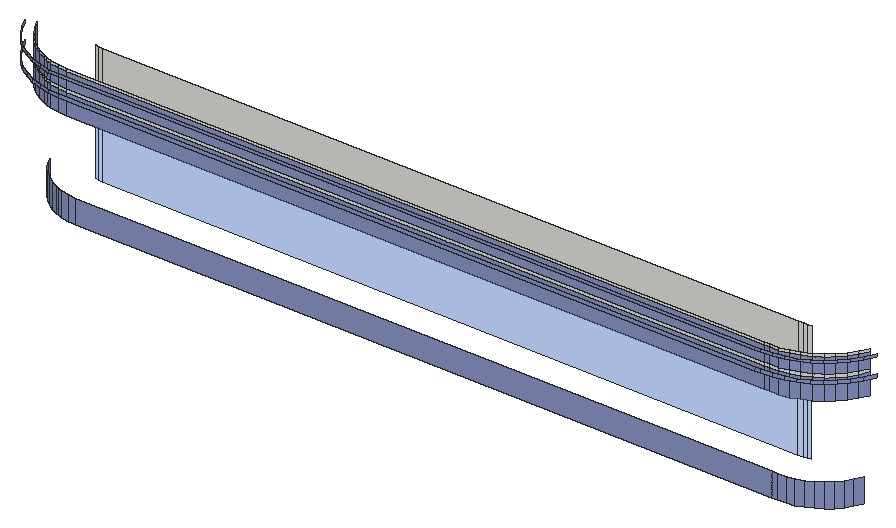
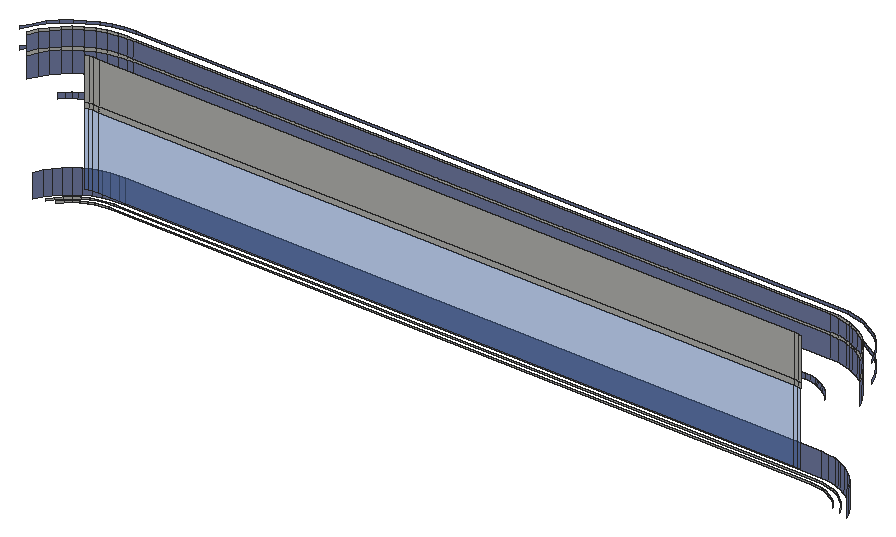
# SketchUp Ruby script. Lengths in inches.
U = 1.inch
M = Sketchup.active_model
def pt(a) = Geom::Point3d.new(a.map { |v| v * U })
def face(e, loops, mat)
  f = e.add_face(loops[0].map { |a| pt(a) })
  loops[1..].each { |l| e.add_face(l.map { |a| pt(a) }).erase! }
  f.material = f.back_material = mat if mat
  f
end
# faces: each face lists its corners as indices into pts; further lists are holes
def faces(e, pts, list, mat = nil) = list.each { |f| face(e, (f[0].is_a?(Array) ? f : [f]).map { |l| l.map { |i| pts[i] } }, mat) }
# xy, xz, yz: faces in a plane at the given z, y or x. An outline is a flat list of corners, or four numbers for a rectangle; further outlines are holes
def ring(l) = l.size == 4 ? [[l[0], l[1]], [l[2], l[1]], [l[2], l[3]], [l[0], l[3]]] : l.each_slice(2).to_a
def flat(e, list, mat, &to3) = list.each { |f| face(e, (f[0].is_a?(Array) ? f : [f]).map { |l| ring(l).map { |u, v| to3.(u, v) } }, mat) }
def xy(e, z, list, mat = nil) = flat(e, list, mat) { |x, y| [x, y, z] }
def xz(e, y, list, mat = nil) = flat(e, list, mat) { |x, z| [x, y, z] }
def yz(e, x, list, mat = nil) = flat(e, list, mat) { |y, z| [x, y, z] }
def lines(e, pts, list) = list.each { |a, b| e.add_line(pt(pts[a]), pt(pts[b])) }
# prism: a flat outline (further loops are holes) pulled along v
def prism(e, loops, v, mat = nil)
  f = face(e, loops, mat); d = Geom::Vector3d.new(v.map { |x| x * U })
  f.pushpull(f.normal.samedirection?(d) ? d.length : -d.length)
end
def box(e, o, s, mat = nil) = prism(e, [[o, [o[0] + s[0], o[1], o[2]], [o[0] + s[0], o[1] + s[1], o[2]], [o[0], o[1] + s[1], o[2]]]], [0, 0, s[2]], mat)
def at(x, y, z, deg = 0) = Geom::Transformation.translation(pt([x, y, z])) * Geom::Transformation.rotation(ORIGIN, Z_AXIS, deg.degrees)
def axes(o, x, y, z) = Geom::Transformation.new([*x, 0, *y, 0, *z, 0, *pt(o).to_a, 1])
def part(name) = M.definitions.add(name)
# library, detail: a bought-in or finely detailed component or shape, given as its bounding box
def library(name, o, s) = part(name).tap { |d| box(d.entities, o, s) }
def detail(e, o, s) = box(e.add_group.entities, o, s)
def put(e, d, t, mat = nil) = e.add_instance(d, t).tap { |i| i.material = mat if mat }
def group(e, t, mat = nil) = e.add_group.tap { |g| g.transformation = t; g.material = mat if mat }.entities
root = M.entities
M.materials.add("0326 AP 7207 CLASSIC PURPLE").color = [140, 152, 201]
M.materials.add("[Translucent Glass Blue]").color = [100, 149, 237]
M.materials["[Translucent Glass Blue]"].alpha = 0.5
xz(root,31.9,[[167.34,433.9375,517.41,435.625],[517.41,433.9375,520.4375,435.625],[167.34,443.3125,517.41,444.625],[517.41,443.3125,520.4375,444.625]],"0326 AP 7207 CLASSIC PURPLE")
xz(root,37.02,[[167.51,433.9375,517.41,435.625],[517.41,433.9375,520.4375,435.625],[167.51,443.3125,517.41,444.625],[517.41,443.3125,520.4375,444.625]])
xz(root,37.02,[[167.51,423.4375,517.41,433.9375],[517.41,423.4375,520.4375,433.9375],[167.51,435.625,517.41,443.3125],[517.41,435.625,520.4375,443.3125]],"0326 AP 7207 CLASSIC PURPLE")
xz(root,42.4375,[[167.6875,372,517.41,384],[517.41,372,520.4375,384]],"0326 AP 7207 CLASSIC PURPLE")
xz(root,45.71,[[167.8,372,517.41,372.8125],[517.41,372,520.4375,372.8125]])
xz(root,48.77,[[167.9,372,517.41,372.8125],[517.41,372,520.4375,372.8125]])
xz(root,52.13,[[168.01,420.75,517.41,423.4375],[517.41,420.75,520.4375,423.4375]],"0326 AP 7207 CLASSIC PURPLE")
xz(root,58.64,[[168.22,420.75,517.41,423.4375],[517.41,420.75,520.4375,423.4375],[168.22,423.4375,517.41,444.625],[517.41,423.4375,520.4375,444.625]])
xz(root,58.64,[[168.22,384,517.41,420.75],[517.41,384,520.4375,420.75]],"[Translucent Glass Blue]")
p = [[167.6875,42.4375,384],[163.74,42.7,384],[163.74,42.7,372],[166.41,42.52,372],[167.6875,42.4375,372],[524.38,42.7,384],
  [520.4375,42.4375,384],[520.4375,42.4375,372],[524.38,42.7,372],[159.87,43.47,384],[159.87,43.47,372],[528.26,43.47,384],
  [528.26,43.47,372],[157.41,44.3,384],[157.41,44.3,372],[532,44.74,384],[532,44.74,372],[156.125,44.74,384],
  [156.125,44.74,372],[152.58,46.49,384],[152.58,46.49,372],[535.55,46.49,384],[535.55,46.49,372],[167.8,45.71,372],
  [166.62,45.78,372],[166.62,45.78,372.8125],[167.8,45.71,372.8125],[523.96,45.9375,372],[520.4375,45.71,372],[520.4375,45.71,372.8125],
  [523.96,45.9375,372.8125],[164.17,45.95,372],[164.17,45.95,372.8125],[160.72,46.63,372],[160.72,46.63,372.8125],[527.41,46.625,372],
  [527.41,46.625,372.8125],[149.29,48.68,384],[149.29,48.68,372],[538.83,48.68,384],[538.83,48.68,372],[158.46,47.4,372],
  [158.46,47.4,372.8125],[530.75,47.76,372],[530.75,47.76,372.8125],[157.38,47.77,372],[157.38,47.77,372.8125],[154.22,49.32,372],
  [154.22,49.32,372.8125],[533.91,49.32,372],[533.91,49.32,372.8125],[146.32,51.29,384],[146.32,51.29,372],[541.81,51.29,384],
  [541.81,51.29,372],[164.57,48.98,372],[166.82,48.84,372],[166.82,48.84,372.8125],[164.57,48.98,372.8125],[167.9,48.77,372],
  [167.9,48.77,372.8125],[520.4375,48.77,372],[523.56,48.97,372],[523.56,48.97,372.8125],[520.4375,48.77,372.8125],[161.51,49.59,372],
  [161.51,49.59,372.8125],[526.62,49.58,372],[526.62,49.58,372.8125],[151.29,51.28,372],[151.29,51.28,372.8125],[536.84,51.28,372],
  [536.84,51.28,372.8125],[159.44,50.3,372],[159.44,50.3,372.8125],[529.58,50.59,372],[529.58,50.59,372.8125],[158.55,50.6,372],
  [158.55,50.6,372.8125],[155.75,51.98,372],[155.75,51.98,372.8125],[532.38,51.97,372],[532.38,51.97,372.8125],[143.71,54.26,384],
  [143.71,54.26,372],[148.64,53.61,372],[148.64,53.61,372.8125],[539.49,53.6,372],[539.49,53.6,372.8125],[544.41,54.26,384],
  [544.41,54.26,372],[153.15,53.71,372],[153.15,53.71,372.8125],[534.98,53.7,372],[534.98,53.7,372.8125],[146.3125,56.26,372],
  [146.3125,56.26,372.8125],[541.82,56.25,372],[541.82,56.25,372.8125],[150.81,55.77,372],[150.81,55.77,372.8125],[537.33,55.76,372],
  [537.33,55.76,372.8125],[141.52,57.55,384],[141.52,57.55,372],[546.61,57.55,384],[546.61,57.55,372],[148.75,58.12,372],
  [148.75,58.12,372.8125],[539.39,58.11,372],[539.39,58.11,372.8125],[144.36,59.1875,372],[144.36,59.1875,372.8125],[543.78,59.18,372],
  [543.78,59.18,372.8125],[139.77,61.09,384],[139.77,61.09,372],[548.36,61.09,384],[548.36,61.09,372],[165.86,58.8,384],
  [168.22,58.64,384],[168.22,58.64,420.75],[165.86,58.8,420.75],[520.4375,58.64,384],[522.27,58.76,384],[522.27,58.76,420.75],
  [520.4375,58.64,420.75],[164.07,59.15,384],[164.07,59.15,420.75],[524.06,59.12,384],[524.06,59.12,420.75],[168.01,52.13,423.4375],
  [165.01,52.33,423.4375],[165.01,52.33,420.75],[168.01,52.13,420.75],[523.12,52.31,423.4375],[520.4375,52.13,423.4375],[520.4375,52.13,420.75],
  [523.12,52.31,420.75],[162.38,52.85,423.4375],[162.38,52.85,420.75],[525.75,52.83,423.4375],[525.75,52.83,420.75],[528.29,53.7,423.4375],
  [528.29,53.7,420.75],[160.52,53.48,423.4375],[160.52,53.48,420.75],[159.84,53.72,423.4375],[159.84,53.72,420.75],[157.4375,54.9,423.4375],
  [157.4375,54.9,420.75],[530.7,54.88,423.4375],[530.7,54.88,420.75],[155.21,56.39,423.4375],[155.21,56.39,420.75],[532.93,56.375,423.4375],
  [532.93,56.375,420.75],[153.19,58.16,423.4375],[153.19,58.16,420.75],[534.95,58.15,423.4375],[534.95,58.15,420.75],[536.72,60.16,423.4375],
  [536.72,60.16,420.75],[151.42,60.18,423.4375],[151.42,60.18,420.75],[168.22,58.64,423.4375],[165.86,58.8,423.4375],[522.27,58.76,423.4375],
  [520.4375,58.64,423.4375],[164.07,59.15,423.4375],[524.06,59.12,423.4375],[163.03,37.3125,423.4375],[167.51,37.02,423.4375],[167.51,37.02,433.9375],
  [163.03,37.3125,433.9375],[520.4375,37.02,423.4375],[525.09,37.32,423.4375],[525.09,37.32,433.9375],[520.4375,37.02,433.9375],[158.46,38.22,423.4375],
  [158.46,38.22,433.9375],[529.66,38.23,423.4375],[529.66,38.23,433.9375],[155.67,39.17,423.4375],[155.67,39.17,433.9375],[534.08,39.73,423.4375],
  [534.08,39.73,433.9375],[154.05,39.72,423.4375],[154.05,39.72,433.9375],[149.86,41.78,423.4375],[149.86,41.78,433.9375],[538.26,41.79,423.4375],
  [538.26,41.79,433.9375],[145.99,44.375,423.4375],[145.99,44.375,433.9375],[542.13,44.38,423.4375],[542.13,44.38,433.9375],[142.48,47.45,423.4375],
  [142.48,47.45,433.9375],[545.64,47.46,423.4375],[545.64,47.46,433.9375],[139.41,50.95,423.4375],[139.41,50.95,433.9375],[548.71,50.96,423.4375],
  [548.71,50.96,433.9375],[136.82,54.83,423.4375],[136.82,54.83,433.9375],[551.3,54.84,423.4375],[551.3,54.84,433.9375],[134.75,59.01,423.4375],
  [134.75,59.01,433.9375],[553.36,59.02,423.4375],[553.36,59.02,433.9375],[165.86,58.8,444.625],[168.22,58.64,444.625],[520.4375,58.64,444.625],
  [522.27,58.76,444.625],[164.07,59.15,444.625],[524.06,59.12,444.625],[162.36,32.22,433.9375],[167.34,31.9,433.9375],[167.34,31.9,435.625],
  [162.36,32.22,435.625],[520.4375,31.9,433.9375],[525.76,32.24,433.9375],[525.76,32.24,435.625],[520.4375,31.9,435.625],[157.13,33.26,433.9375],
  [157.13,33.26,435.625],[530.99,33.28,433.9375],[530.99,33.28,435.625],[154.02,34.32,433.9375],[154.02,34.32,435.625],[536.04,35,433.9375],
  [536.04,35,435.625],[152.08,34.98,433.9375],[152.08,34.98,435.625],[147.3,37.34,433.9375],[147.3,37.34,435.625],[540.82,37.36,433.9375],
  [540.82,37.36,435.625],[163.03,37.3125,435.625],[167.51,37.02,435.625],[520.4375,37.02,435.625],[525.09,37.32,435.625],[142.86,40.3,433.9375],
  [142.86,40.3,435.625],[158.46,38.22,435.625],[529.66,38.23,435.625],[545.25,40.32,433.9375],[545.25,40.32,435.625],[155.67,39.17,435.625],
  [534.08,39.73,435.625],[154.05,39.72,435.625],[149.86,41.78,435.625],[538.26,41.79,435.625],[138.85,43.82,433.9375],[138.85,43.82,435.625],
  [549.26,43.83,433.9375],[549.26,43.83,435.625],[145.99,44.375,435.625],[542.13,44.38,435.625],[135.33,47.83,433.9375],[135.33,47.83,435.625],
  [552.78,47.84,433.9375],[552.78,47.84,435.625],[142.48,47.45,435.625],[545.64,47.46,435.625],[139.41,50.95,435.625],[548.71,50.96,435.625],
  [132.37,52.26,433.9375],[132.37,52.26,435.625],[555.74,52.28,433.9375],[555.74,52.28,435.625],[136.82,54.83,435.625],[551.3,54.84,435.625],
  [130.01,57.05,433.9375],[130.01,57.05,435.625],[558.1,57.06,433.9375],[558.1,57.06,435.625],[134.75,59.01,435.625],[553.36,59.02,435.625],
  [167.51,37.02,443.3125],[163.03,37.3125,443.3125],[525.09,37.32,443.3125],[520.4375,37.02,443.3125],[158.46,38.22,443.3125],[529.66,38.23,443.3125],
  [155.67,39.17,443.3125],[534.08,39.73,443.3125],[154.05,39.72,443.3125],[149.86,41.78,443.3125],[538.26,41.79,443.3125],[145.99,44.375,443.3125],
  [542.13,44.38,443.3125],[142.48,47.45,443.3125],[545.64,47.46,443.3125],[139.41,50.95,443.3125],[548.71,50.96,443.3125],[136.82,54.83,443.3125],
  [551.3,54.84,443.3125],[134.75,59.01,443.3125],[553.36,59.02,443.3125],[162.36,32.22,443.3125],[167.34,31.9,443.3125],[167.34,31.9,444.625],
  [162.36,32.22,444.625],[520.4375,31.9,443.3125],[525.76,32.24,443.3125],[525.76,32.24,444.625],[520.4375,31.9,444.625],[157.13,33.26,443.3125],
  [157.13,33.26,444.625],[530.99,33.28,443.3125],[530.99,33.28,444.625],[154.02,34.32,443.3125],[154.02,34.32,444.625],[536.04,35,443.3125],
  [536.04,35,444.625],[152.08,34.98,443.3125],[152.08,34.98,444.625],[147.3,37.34,443.3125],[147.3,37.34,444.625],[540.82,37.36,443.3125],
  [540.82,37.36,444.625],[163.03,37.3125,444.625],[167.51,37.02,444.625],[520.4375,37.02,444.625],[525.09,37.32,444.625],[142.86,40.3,443.3125],
  [142.86,40.3,444.625],[158.46,38.22,444.625],[529.66,38.23,444.625],[545.25,40.32,443.3125],[545.25,40.32,444.625],[155.67,39.17,444.625],
  [534.08,39.73,444.625],[154.05,39.72,444.625],[149.86,41.78,444.625],[538.26,41.79,444.625],[138.85,43.82,443.3125],[138.85,43.82,444.625],
  [549.26,43.83,443.3125],[549.26,43.83,444.625],[145.99,44.375,444.625],[542.13,44.38,444.625],[135.33,47.83,443.3125],[135.33,47.83,444.625],
  [552.78,47.84,443.3125],[552.78,47.84,444.625],[142.48,47.45,444.625],[545.64,47.46,444.625],[139.41,50.95,444.625],[548.71,50.96,444.625],
  [132.37,52.26,443.3125],[132.37,52.26,444.625],[555.74,52.28,443.3125],[555.74,52.28,444.625],[136.82,54.83,444.625],[551.3,54.84,444.625],
  [130.01,57.05,443.3125],[130.01,57.05,444.625],[558.1,57.06,443.3125],[558.1,57.06,444.625],[134.75,59.01,444.625],[553.36,59.02,444.625]]
faces(root,p,[[0,1,2,3,4],[5,6,7,8],[1,9,10,2],[11,5,8,12],[9,13,14,10],[15,11,12,16],[13,17,18,14],[17,19,20,18],
  [21,15,16,22],[19,37,38,20],[39,21,22,40],[37,51,52,38],[53,39,40,54],[51,83,84,52],[89,53,54,90],[83,103,104,84],
  [105,89,90,106],[103,115,116,104],[117,105,106,118],[131,132,133,134],[135,136,137,138],[132,139,140,133],[141,135,138,142],[143,141,142,144],
  [139,145,146,140],[145,147,148,146],[147,149,150,148],[151,143,144,152],[149,153,154,150],[155,151,152,156],[153,157,158,154],[159,155,156,160],
  [161,159,160,162],[157,163,164,158],[171,172,173,174],[175,176,177,178],[179,171,174,180],[176,181,182,177],[183,179,180,184],[181,185,186,182],
  [187,183,184,188],[189,187,188,190],[185,191,192,186],[193,189,190,194],[191,195,196,192],[197,193,194,198],[195,199,200,196],[201,197,198,202],
  [199,203,204,200],[205,201,202,206],[203,207,208,204],[209,205,206,210],[207,211,212,208],[219,220,221,222],[223,224,225,226],[227,219,222,228],
  [224,229,230,225],[231,227,228,232],[229,233,234,230],[235,231,232,236],[237,235,236,238],[233,239,240,234],[245,237,238,246],[239,249,250,240],
  [256,245,246,257],[249,258,259,250],[262,256,257,263],[258,264,265,259],[270,262,263,271],[264,272,273,265],[276,270,271,277],[272,278,279,273],
  [241,242,282,283],[243,244,284,285],[247,241,283,286],[244,248,287,284],[251,247,286,288],[248,252,289,287],[253,251,288,290],[254,253,290,291],
  [252,255,292,289],[260,254,291,293],[255,261,294,292],[266,260,293,295],[261,267,296,294],[268,266,295,297],[267,269,298,296],[274,268,297,299],
  [269,275,300,298],[280,274,299,301],[275,281,302,300],[303,304,305,306],[307,308,309,310],[311,303,306,312],[308,313,314,309],[315,311,312,316],
  [313,317,318,314],[319,315,316,320],[321,319,320,322],[317,323,324,318],[329,321,322,330],[323,333,334,324],[340,329,330,341],[333,342,343,334],
  [346,340,341,347],[342,348,349,343],[354,346,347,355],[348,356,357,349],[360,354,355,361],[356,362,363,357]],"0326 AP 7207 CLASSIC PURPLE")
faces(root,p,[[23,24,25,26],[27,28,29,30],[24,31,32,25],[31,33,34,32],[35,27,30,36],[33,41,42,34],[43,35,36,44],[41,45,46,42],
  [45,47,48,46],[49,43,44,50],[55,56,57,58],[56,59,60,57],[61,62,63,64],[65,55,58,66],[62,67,68,63],[47,69,70,48],
  [71,49,50,72],[73,65,66,74],[67,75,76,68],[77,73,74,78],[79,77,78,80],[75,81,82,76],[69,85,86,70],[87,71,72,88],
  [91,79,80,92],[81,93,94,82],[85,95,96,86],[97,87,88,98],[99,91,92,100],[93,101,102,94],[107,99,100,108],[101,109,110,102],
  [95,111,112,96],[113,97,98,114],[165,166,122,121],[167,168,126,125],[166,169,128,122],[170,167,125,130],[165,166,213,214],[167,168,215,216],
  [166,169,217,213],[170,167,216,218],[173,174,241,242],[177,178,243,244],[174,180,247,241],[182,177,244,248],[180,184,251,247],[186,182,248,252],
  [184,188,253,251],[188,190,254,253],[192,186,252,255],[190,194,260,254],[196,192,255,261],[194,198,266,260],[200,196,261,267],[198,202,268,266],
  [204,200,267,269],[202,206,274,268],[208,204,269,275],[206,210,280,274],[212,208,275,281],[282,283,325,326],[284,285,327,328],[283,286,331,325],
  [287,284,328,332],[286,288,335,331],[289,287,332,336],[288,290,337,335],[290,291,338,337],[292,289,336,339],[291,293,344,338],[294,292,339,345],
  [293,295,350,344],[296,294,345,351],[295,297,352,350],[298,296,351,353],[297,299,358,352],[300,298,353,359],[299,301,364,358],[302,300,359,365]])
faces(root,p,[[119,120,121,122],[123,124,125,126],[127,119,122,128],[124,129,130,125]],"[Translucent Glass Blue]")
